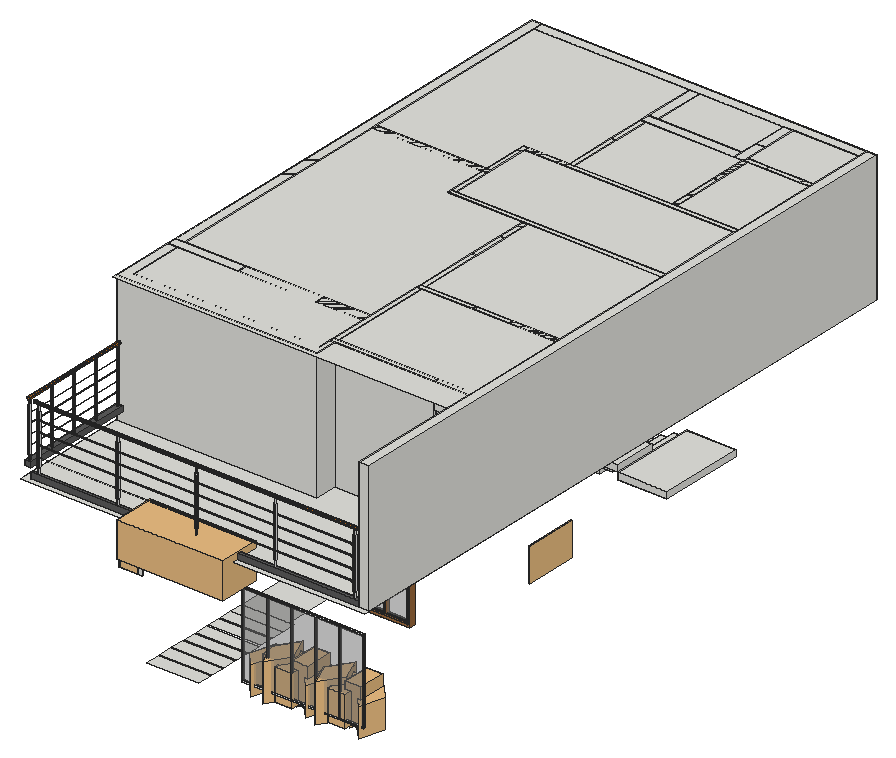
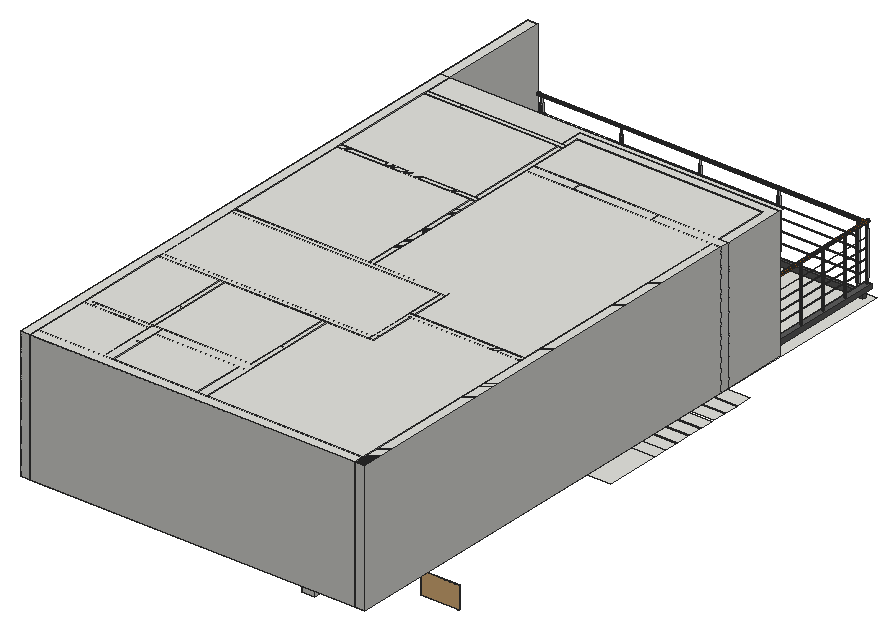
# SketchUp Ruby script. Lengths in inches.
U = 1.inch
M = Sketchup.active_model
def pt(a) = Geom::Point3d.new(a.map { |v| v * U })
def face(e, loops, mat)
  f = e.add_face(loops[0].map { |a| pt(a) })
  loops[1..].each { |l| e.add_face(l.map { |a| pt(a) }).erase! }
  f.material = f.back_material = mat if mat
  f
end
# faces: each face lists its corners as indices into pts; further lists are holes
def faces(e, pts, list, mat = nil) = list.each { |f| face(e, (f[0].is_a?(Array) ? f : [f]).map { |l| l.map { |i| pts[i] } }, mat) }
# xy, xz, yz: faces in a plane at the given z, y or x. An outline is a flat list of corners, or four numbers for a rectangle; further outlines are holes
def ring(l) = l.size == 4 ? [[l[0], l[1]], [l[2], l[1]], [l[2], l[3]], [l[0], l[3]]] : l.each_slice(2).to_a
def flat(e, list, mat, &to3) = list.each { |f| face(e, (f[0].is_a?(Array) ? f : [f]).map { |l| ring(l).map { |u, v| to3.(u, v) } }, mat) }
def xy(e, z, list, mat = nil) = flat(e, list, mat) { |x, y| [x, y, z] }
def xz(e, y, list, mat = nil) = flat(e, list, mat) { |x, z| [x, y, z] }
def yz(e, x, list, mat = nil) = flat(e, list, mat) { |y, z| [x, y, z] }
def lines(e, pts, list) = list.each { |a, b| e.add_line(pt(pts[a]), pt(pts[b])) }
# prism: a flat outline (further loops are holes) pulled along v
def prism(e, loops, v, mat = nil)
  f = face(e, loops, mat); d = Geom::Vector3d.new(v.map { |x| x * U })
  f.pushpull(f.normal.samedirection?(d) ? d.length : -d.length)
end
def box(e, o, s, mat = nil) = prism(e, [[o, [o[0] + s[0], o[1], o[2]], [o[0] + s[0], o[1] + s[1], o[2]], [o[0], o[1] + s[1], o[2]]]], [0, 0, s[2]], mat)
def at(x, y, z, deg = 0) = Geom::Transformation.translation(pt([x, y, z])) * Geom::Transformation.rotation(ORIGIN, Z_AXIS, deg.degrees)
def axes(o, x, y, z) = Geom::Transformation.new([*x, 0, *y, 0, *z, 0, *pt(o).to_a, 1])
def part(name) = M.definitions.add(name)
# library, detail: a bought-in or finely detailed component or shape, given as its bounding box
def library(name, o, s) = part(name).tap { |d| box(d.entities, o, s) }
def detail(e, o, s) = box(e.add_group.entities, o, s)
def put(e, d, t, mat = nil) = e.add_instance(d, t).tap { |i| i.material = mat if mat }
def group(e, t, mat = nil) = e.add_group.tap { |g| g.transformation = t; g.material = mat if mat }.entities
root = M.entities
M.materials.add("JJJ1").color = [238, 218, 183]
M.materials.add("MU TIGHI 6T67L 1").color = [235, 235, 235]
M.materials.add("Polis06_194").color = [79, 50, 36]
M.materials.add("Stone_A_200cm").color = [133, 133, 133]
M.materials.add("T ER5Y 565N 1").color = [201, 111, 22]
M.materials.add("T R72 56 8, 7 5U1").color = [25, 25, 25]
M.materials.add("[Color M00]").color = [255, 255, 255]
M.materials.add("[Color M09]").color = [0, 0, 0]
M.materials.add("[Translucent Glass Gray]").color = [128, 128, 128]
M.materials["[Translucent Glass Gray]"].alpha = 0.5
M.materials.add("[Translucent Glass Gray]1").color = [128, 128, 128]
M.materials["[Translucent Glass Gray]1"].alpha = 0.29
M.materials.add("[Translucent_Glass_Gray]").color = [128, 128, 128]
M.materials["[Translucent_Glass_Gray]"].alpha = 0.5
M.materials.add("[Wood Floor]").color = [155, 105, 61]
M.materials.add("wefsd tger 1").color = [92, 92, 92]
c1 = library("Group\#103",[-84.69,-90.07,-0.36],[176.51,175.13,171.4])
c2 = library("Areca palm plant",[0,0,0],[49.1,36.6,54.46])
c3 = part("Group\#23")
box(c3.entities,[0,0,0],[12.05,39.48,6])
c4 = library("Group\#130",[-7.34,-1.2,0],[38.67,35.81,49.04])
c5 = library("Group20\#1",[-20.81,-17.08,3.79],[39.86,39.43,37.51])
c6 = library("Group38\#2",[14.01,28.44,-23.43],[18.58,18.32,38.89])
c7 = part("W1")
xy(c7.entities,15,[[0,0,2,198]])
xy(c7.entities,102.0625,[[0,0,2,198]],"[Color M00]")
xz(c7.entities,0,[[0,15,2,102.0625]],"[Color M00]")
xz(c7.entities,198,[[0,15,2,102.0625]])
yz(c7.entities,0,[[0.84,16,39.43,101.0625],[40.28,16,78.87,101.0625],[79.71,16,118.3,101.0625],[119.14,16,157.73,101.0625],[158.58,16,197.16,101.0625]])
yz(c7.entities,0,[[[0,15,198,102.0625],[0.84,16,197.16,101.0625]],[39.43,16,40.28,101.0625],[78.87,16,79.71,101.0625],[118.3,16,119.14,101.0625],[157.73,16,158.58,101.0625]],"[Color M00]")
yz(c7.entities,2,[[0.84,16,39.43,101.0625],[40.28,16,78.87,101.0625],[79.71,16,118.3,101.0625],[119.14,16,157.73,101.0625],[158.58,16,197.16,101.0625]])
yz(c7.entities,2,[[[0,15,198,102.0625],[0.84,16,197.16,101.0625]],[39.43,16,40.28,101.0625],[78.87,16,79.71,101.0625],[118.3,16,119.14,101.0625],[157.73,16,158.58,101.0625]],"[Color M00]")
c8 = part("window full")
xy(c8.entities,0,[[0,0,14.17,66.54]])
xy(c8.entities,2.26,[[12.2,2.26,14.17,64.28]],"[Wood Floor]")
xy(c8.entities,2.36,[[0,2.36,1.97,64.17]],"[Wood Floor]")
xy(c8.entities,3.74,[[11.42,3.74,12.2,32.875],[11.42,33.66,12.2,62.79]],"[Wood Floor]")
xy(c8.entities,3.9375,[[1.97,3.9375,2.76,32.77],[1.97,33.76,2.76,62.6]],"[Wood Floor]")
xy(c8.entities,4.18,[[2.76,4.18,7.09,32.09],[7.09,4.18,11.42,32.09],[2.76,34.45,7.09,62.35],[7.09,34.45,11.42,62.35]],"[Wood Floor]")
xy(c8.entities,69.83,[[2.76,4.18,7.09,32.09],[7.09,32.09,11.42,34.45],[2.76,34.45,7.09,62.35]])
xy(c8.entities,69.83,[[7.09,4.18,11.42,32.09],[7.09,34.45,11.42,62.35]],"[Wood Floor]")
xy(c8.entities,70.08,[[1.97,3.9375,2.76,32.77],[1.97,33.76,2.76,62.6]])
xy(c8.entities,70.27,[[11.42,32.875,12.2,33.66]])
xy(c8.entities,70.27,[[11.42,3.74,12.2,32.875],[11.42,33.66,12.2,62.79]],"[Wood Floor]")
xy(c8.entities,71.65,[[0,2.36,1.97,64.17]])
xy(c8.entities,71.76,[[12.2,2.26,14.17,64.28]],"[Wood Floor]")
xy(c8.entities,74.02,[[0,0,14.17,66.54]],"[Wood Floor]")
xz(c8.entities,0,[[0,0,14.17,74.02]],"[Wood Floor]")
xz(c8.entities,2.26,[[12.2,2.26,14.17,71.76]],"[Wood Floor]")
xz(c8.entities,2.36,[[0,2.36,1.97,71.65]],"[Wood Floor]")
xz(c8.entities,3.74,[[11.42,3.74,12.2,70.27]],"[Wood Floor]")
xz(c8.entities,3.9375,[[1.97,3.9375,2.76,70.08]],"[Wood Floor]")
xz(c8.entities,4.18,[[2.76,4.18,7.09,69.83],[7.09,4.18,11.42,69.83]],"[Wood Floor]")
xz(c8.entities,32.09,[[2.76,4.18,11.42,69.83]],"[Wood Floor]")
xz(c8.entities,32.77,[[1.97,3.9375,2.76,70.08]],"[Wood Floor]")
xz(c8.entities,32.875,[[11.42,3.74,12.2,70.27]],"[Wood Floor]")
xz(c8.entities,33.66,[[11.42,3.74,12.2,47.88],[11.42,47.88,12.2,70.27]],"[Wood Floor]")
xz(c8.entities,33.76,[[1.97,3.9375,2.76,70.08]],"[Wood Floor]")
xz(c8.entities,34.45,[[2.76,4.18,11.42,69.83]],"[Wood Floor]")
xz(c8.entities,62.35,[[2.76,4.18,7.09,69.83],[7.09,4.18,11.42,69.83]],"[Wood Floor]")
xz(c8.entities,62.6,[[1.97,3.9375,2.76,70.08]],"[Wood Floor]")
xz(c8.entities,62.79,[[11.42,3.74,12.2,70.27]],"[Wood Floor]")
xz(c8.entities,64.17,[[0,2.36,1.97,71.65]],"[Wood Floor]")
xz(c8.entities,64.28,[[12.2,2.26,14.17,71.76]],"[Wood Floor]")
xz(c8.entities,66.54,[[0,0,14.17,74.02]],"[Wood Floor]")
yz(c8.entities,0,[[[0,0,66.54,74.02],[2.36,2.36,64.17,71.65]]],"[Wood Floor]")
yz(c8.entities,1.97,[[[2.36,2.36,64.17,71.65],[33.76,3.9375,62.6,70.08],[3.9375,3.9375,32.77,70.08]]],"[Wood Floor]")
yz(c8.entities,2.76,[[32.77,3.9375,33.76,4.18],[32.77,4.18,33.76,69.83],[32.77,69.83,33.76,70.08]])
yz(c8.entities,2.76,[[[3.9375,3.9375,32.77,70.08],[4.18,4.18,32.09,69.83]],[[33.76,3.9375,62.6,70.08],[34.45,4.18,62.35,69.83]]],"[Wood Floor]")
yz(c8.entities,7.09,[[4.18,4.18,62.35,69.83]],"[Translucent Glass Gray]")
yz(c8.entities,11.42,[[32.875,69.83,33.66,70.27]])
yz(c8.entities,11.42,[[[3.74,3.74,32.875,70.27],[4.18,4.18,32.09,69.83]],[[33.66,3.74,62.79,70.27],[34.45,4.18,62.35,69.83]]],"[Wood Floor]")
yz(c8.entities,12.2,[[[2.26,2.26,64.28,71.76],[3.74,3.74,32.875,70.27],[33.66,3.74,62.79,70.27]]],"[Wood Floor]")
yz(c8.entities,14.17,[[[0,0,66.54,74.02],[2.26,2.26,64.28,71.76]]],"[Wood Floor]")
p = [[11.42,32.875,70.27],[11.42,32.875,70.28]]
lines(c8.entities,p,[[0,1]])
c9 = library("Flat screen television",[0,1.41,1.14],[35.92,0.28,20.21])
c10 = library("TempSimLab_2015-06-11-13-14-41",[-24.54,-1.375,2.18],[48.7,1.34,30.98])
c11 = part("Group\#54")
prism(c11.entities,[[[0,39.5,0],[12,39.52,0],[12.05,0.02,0],[0.05,0,0]]],[0,0,6])
c12 = library("B_HOUSE",[0,0,0],[67.64,11.09,0.98])
c13 = library("Group\#92",[-9.3,-11.72,-5.59],[177.13,38.12,35])
c14 = part("Component\#28")
box(c14.entities,[0,0,0],[7.875,7.875,3.9375],"Stone_A_200cm")
c15 = part("Flush door")
xy(c15.entities,0,[[0,0,4.72,1.18],[0,34.25,4.72,35.43]],"Polis06_194")
xy(c15.entities,85.26,[[0,1.18,4.72,34.25]],"Polis06_194")
xy(c15.entities,86.61,[[0,0,4.72,35.43]],"Polis06_194")
xz(c15.entities,0,[[0,0,4.72,86.61]],"Polis06_194")
xz(c15.entities,1.18,[[0,0,2.36,85.26],[2.36,0,4.72,85.26]],"Polis06_194")
xz(c15.entities,34.25,[[0,0,4.72,85.26]],"Polis06_194")
xz(c15.entities,35.43,[[0,0,4.72,86.61]],"Polis06_194")
yz(c15.entities,0,[[0,0,1.18,86.61],[34.25,0,35.43,86.61],[1.18,85.26,34.25,86.61]],"Polis06_194")
yz(c15.entities,2.36,[[1.18,0,34.25,0,34.25,85.21,1.18,85.26]],"Polis06_194")
yz(c15.entities,4.72,[[0,0,1.18,86.61],[34.25,0,35.43,86.61],[1.18,85.26,34.25,86.61]],"Polis06_194")
c16 = part("Group\#68")
p = [[0,43.31,5.11],[2.95,43.31,0],[2.95,0,0],[0,0,5.11]]
faces(c16.entities,p,[[0,1,2,3]],"[Translucent_Glass_Gray]")
c17 = part("Vwntilation+window (2)")
put(c17.entities,c16,at(43.48,1.97,32.29))
put(c17.entities,c16,at(43.48,1.97,26.38))
put(c17.entities,c16,at(43.48,1.97,20.48))
put(c17.entities,c16,at(43.48,1.97,14.57))
put(c17.entities,c16,at(43.48,1.97,8.67))
put(c17.entities,c16,at(43.48,1.97,2.76))
g1 = group(c17.entities,at(43.48,0,0))
prism(g1,[[[1.97,47.24,39.37],[1.97,0,39.37],[1.97,0,0],[1.97,47.24,0]],[[1.97,45.28,1.97],[1.97,1.97,1.97],[1.97,1.97,37.4],[1.97,45.28,37.4]]],[-1.97,0,0])
c18 = part("Box01")
box(c18.entities,[-251.12,-5.93,-8.91],[582.61,12.27,8.91],"wefsd tger 1")
c19 = part("Box45")
box(c19.entities,[-240.91,-0.82,12.1],[2.44,1.82,74.48],"JJJ1")
c20 = part("Cylinder01")
prism(c20.entities,[[[328.21,-1.16,98.56],[328.21,-0.34,98.26],[328.21,0.53,98.26],[328.21,1.34,98.56],[328.21,2.01,99.11],[328.21,2.44,99.87],[328.21,2.59,100.72],[328.21,2.44,101.58],[328.21,2.01,102.33],[328.21,1.34,102.89],[328.21,0.53,103.18],[328.21,-0.34,103.18],[328.21,-1.16,102.89],[328.21,-1.82,102.33],[328.21,-2.25,101.58],[328.21,-2.41,100.72],[328.21,-2.25,99.87],[328.21,-1.82,99.11]]],[-576.3,0,0],"T ER5Y 565N 1")
c21 = part("Cylinder02")
prism(c21.entities,[[[-239.93,0.18,76.32],[-239.93,0.34,76.26],[-239.93,0.48,76.15],[-239.93,0.5625,75.99],[-239.93,0.59,75.82],[-239.93,0.5625,75.65],[-239.93,0.48,75.5],[-239.93,0.34,75.39],[-239.93,0.18,75.33],[-239.93,0.01,75.33],[-239.93,-0.16,75.39],[-239.93,-0.29,75.5],[-239.93,-0.375,75.65],[-239.93,-0.41,75.82],[-239.93,-0.375,75.99],[-239.93,-0.29,76.15],[-239.93,-0.16,76.26],[-239.93,0.01,76.32]]],[560.05,0,0],"T R72 56 8, 7 5U1")
c22 = part("Rectangle1")
prism(c22.entities,[[[-237.41,1.91,10.08],[-239.22,1.91,10.08],[-239.22,1.91,0.02],[-240.41,1.91,0.02],[-240.41,1.91,10.08],[-242.22,1.91,10.08],[-242.22,1.91,89.41],[-240.41,1.91,89.41],[-240.41,1.91,99.1875],[-239.22,1.91,99.1875],[-239.22,1.91,89.41],[-237.41,1.91,89.41]],[[-240.4375,1.91,85.68],[-240.4375,1.91,13.53],[-239.08,1.91,13.53],[-239.08,1.91,85.68]]],[0,-3.64,0],"MU TIGHI 6T67L 1")
c23 = part("skp243")
put(c23.entities,c18,at(0,0,0))
put(c23.entities,c19,at(0,0,0))
put(c23.entities,c20,at(0,0,0))
put(c23.entities,c21,at(0,0,0))
put(c23.entities,c22,at(0,0,0))
put(c23.entities,c21,at(0,0,-17.07))
put(c23.entities,c21,at(0,0,-35.38))
put(c23.entities,c21,at(0,0,-53.15))
put(c23.entities,c19,at(139.83,0,0))
put(c23.entities,c22,at(139.83,0,0))
put(c23.entities,c22,at(279.78,0,0))
put(c23.entities,c19,at(279.78,0,0))
put(c23.entities,c19,at(419.57,0,0))
put(c23.entities,c22,at(419.57,0,0))
put(c23.entities,c22,at(561.11,0,0))
put(c23.entities,c19,at(561.11,0,0))
c24 = part("Railing1 (1)")
put(c24.entities,c23,at(251.12,5.93,8.91))
c25 = part("Group\#49")
box(c25.entities,[0,0,0],[12.05,39.33,6])
xy(root,2,[[138.47,57,186.47,70.5],[138.47,72.5,186.47,84.5],[138.47,86.5,186.47,98.5],[138.47,100.5,186.47,112.5],[138.47,114.5,186.47,126.5],
  [138.47,128.5,186.47,140.5],[138.47,142.5,186.47,154.5],[138.47,154.5,186.47,166.5],[138.47,166.5,181.66,218]])
xy(root,120,[[28.97,48,346.97,638.5]])
put(root,c1,axes([304.91,79.66,5.45],[-0.04107,0.04465,0],[-0.02371,-0.07734,0],[0,0,0.0947]))
put(root,c1,axes([314.5,79.66,5.45],[-0.04107,0.04465,0],[-0.02371,-0.07734,0],[0,0,0.0947]))
put(root,c1,axes([291.89,79.66,5.45],[-0.04107,0.04465,0],[-0.02371,-0.07734,0],[0,0,0.0947]))
put(root,c1,axes([243.23,79.66,5.45],[-0.04107,0.04465,0],[-0.02371,-0.07734,0],[0,0,0.0947]))
put(root,c1,axes([256.25,79.66,5.45],[-0.04107,0.04465,0],[-0.02371,-0.07734,0],[0,0,0.0947]))
put(root,c1,axes([265.84,79.66,5.45],[-0.04107,0.04465,0],[-0.02371,-0.07734,0],[0,0,0.0947]))
put(root,c1,axes([280.11,77.63,5.47],[-0.06732,0.0732,0],[-0.03887,-0.12678,0],[0,0,0.15525]))
put(root,c1,axes([229.72,77.63,5.47],[-0.06732,0.0732,0],[-0.03887,-0.12678,0],[0,0,0.15525]))
put(root,c1,axes([328.77,77.63,5.47],[-0.06732,0.0732,0],[-0.03887,-0.12678,0],[0,0,0.15525]))
put(root,c2,axes([297.88,98.68,5.48],[-0.26854,-0.40516,0],[0.25322,-0.59523,0],[0,0,0.648]))
put(root,c2,axes([249.22,98.68,5.48],[-0.26854,-0.40516,0],[0.25322,-0.59523,0],[0,0,0.648]))
put(root,c3,at(196.65,447.38,6))
put(root,c4,axes([265.14,70.66,7.2],[0.37755,0,0],[0,0.711,0],[0,0,0.711]))
put(root,c4,axes([313.8,70.66,7.2],[0.37755,0,0],[0,0.711,0],[0,0,0.711]))
put(root,c5,axes([260.4,76.03,4.3],[0.40622,0,0],[0,0.765,0],[0,0,0.765]))
put(root,c5,axes([309.05,76.03,4.3],[0.40622,0,0],[0,0.765,0],[0,0,0.765]))
put(root,c6,axes([221.625,96.8,25.35],[0,-0.79632,0],[0.45245,0,0],[0,0,0.77243]))
put(root,c6,axes([270.28,96.8,25.35],[0,-0.79632,0],[0.45245,0,0],[0,0,0.77243]))
put(root,c3,at(208.7,447.38,12))
put(root,c7,axes([222.18,64.3,0],[0,-0.9,0],[0.56673,0,0],[0,0,0.9]),"[Translucent Glass Gray]1")
put(root,c3,at(220.75,447.38,18))
put(root,c3,at(232.8,447.38,24))
put(root,c3,at(244.85,447.38,30))
put(root,c8,axes([291.92,168.52,36],[0,0.4275,0],[-0.72142,0,0],[0,0,0.64851]))
put(root,c3,at(256.9,447.38,36))
put(root,c3,at(268.95,447.38,42))
put(root,c9,at(188.82,267,42.23,90))
put(root,c9,at(94.34,493.52,45.0625,180))
put(root,c3,at(281,447.38,48))
put(root,c10,at(338.01,274.3125,50.51,-90))
g2 = group(root,at(293.05,407.86,54))
box(g2,[0,0,0],[45.375,79,6])
put(root,c11,at(281,407.86,60))
put(root,c11,at(269,407.86,66))
put(root,c11,at(257,407.86,72))
g3 = group(root,at(146.24,51.15,76.77))
box(g3,[-28.68,0,0],[21.64,0.79,11.8125])
put(root,c12,axes([118.79,51.15,77.42],[0.24123,0,0],[0,0,0.9088],[0,-0.64,0]),"[Color M09]")
put(root,c11,at(245,407.86,78))
put(root,c11,at(233,407.86,84))
put(root,c11,at(221,407.86,90))
put(root,c13,axes([132.7,48,98.23],[0.55,0,0],[0,1,0],[0,0,0.94148]))
put(root,c11,at(209,407.86,96))
g4 = group(root,at(115.85,487,0))
box(g4,[0,0,96],[40,4.5,24])
g5 = group(root,at(273.47,493.55,0))
box(g5,[0,0,96],[4.5,32.16,24])
put(root,c14,axes([140.28,49.97,100.39],[0.55,0,0],[0,1,0],[0,0,1]))
put(root,c14,axes([216.08,49.97,100.39],[0.55,0,0],[0,1,0],[0,0,1]))
put(root,c11,at(197,407.86,102))
put(root,c11,at(185,407.85,108))
g6 = group(root,at(28.97,53,120))
xy(g6,0,[[[0,0,309,576.5],[153,437.37,157.5,437.5]],[153,437.37,157.5,437.5]])
xy(g6,120,[[0,101.55,318,585.5]])
put(g6,c15,axes([111.86,354.25,0],[0.7,0,0],[0,1.00894,0],[0,0,1.10836]))
put(g6,c15,axes([111.86,430.25,0],[0.7,0,0],[0,-1.00894,0],[0,0,1.10836]))
put(g6,c15,axes([300.53,519.5,0],[0,0.7,0],[-0.9075,0,0],[0,0,1.10836]))
put(g6,c17,axes([277,179.91,60],[0,-1.16,0],[0.67733,0,0],[0,0,0.92]))
put(g6,c17,axes([197.55,544.5,60],[1,0,0],[0,0.67733,0],[0,0,1]))
put(g6,c8,axes([137.1875,165,36],[0,0.4275,0],[-1.08213,0,0],[0,0,0.64851]))
put(g6,c15,axes([247.5,485.52,0],[0.7,0,0],[0,0.9075,0],[0,0,1.10836]))
put(g6,c15,axes([153,485.52,0],[0.7,0,0],[0,0.9075,0],[0,0,1.10836]))
put(g6,c15,axes([180.5,290.47,0],[0.7,0,0],[0,0.9075,0],[0,0,1.10836]))
put(g6,c15,axes([265.35,227,0],[0,0.7,0],[-0.9075,0,0],[0,0,1.10836]))
put(g6,c24,axes([6.04,0,0],[0.52,0,0],[0,0.26,0],[0,0,0.58]))
put(g6,c24,axes([0,106,8.91],[0,-0.18194,0],[0.49244,0,0],[0,0,0.51123]))
g7 = group(g6,at(0,106,0))
prism(g7,[[[185,0,0],[0,0,0],[0,59,0],[9,59,0],[9,9,0],[180.5,9,0],[180.5,20.5,0],[185,20.5,0]]],[0,0,120])
g8 = group(g6,at(65.1875,165,0))
box(g8,[0,0,0],[72,9,36])
box(g8,[0,0,84],[72,9,36])
p = [[0,9,36],[0,9,84],[72,9,36],[72,9,84]]
lines(g8,p,[[0,1],[2,3]])
g9 = group(g6,at(180.5,126.5,0))
prism(g9,[[[4.5,0,0],[0,0,0],[0,4.5,0],[4.5,4.5,0],[96.5,4.5,0],[96.5,0,0]]],[0,0,120])
g10 = group(g6,at(9,390,0))
box(g10,[0,0,0],[106.17,4.5,120])
g11 = group(g6,at(0,165,0))
prism(g11,[[[65.1875,9,0],[65.1875,0,0],[9,0,0],[0,0,0],[0,9,0],[9,9,0]]],[0,0,120])
g12 = group(g6,at(137.1875,165,0))
box(g12,[0,0,0],[43.3125,9,120])
g13 = group(g6,at(239.5,519.5,0))
prism(g13,[[[9,4.5,0],[9,0,0],[0,0,0],[0,8.85,0],[0,25,0],[9,25,0]]],[0,0,120])
g14 = group(g6,at(153,519.5,0))
box(g14,[0,0,0],[86.5,8.85,120])
g15 = group(g6,at(153,528.5,0))
box(g15,[0,0,0],[9,48,120])
g16 = group(g6,at(309,0,0))
prism(g16,[[[0,576.5,0],[0,585.5,0],[9,585.5,0],[9,0,0],[0,0,0],[0,126.5,0],[0,131,0],[0,227,0],[0,231.5,0],[0,349.55,0],[0,354,0],[0,432.8125,0],[0,437.5,0],[0,519.5,0],[0,524,0]]],[0,0,120])
g17 = group(g6,at(247.5,437.5,0))
box(g17,[0,0,0],[4.5,48.02,120])
g18 = group(g6,at(153,437.5,0))
box(g18,[0,0,0],[4.5,48.02,120])
g19 = group(g6,at(180.5,131,0))
prism(g19,[[[0,0,0],[0,34,0],[0,43,0],[0,96,0],[4.5,96,0],[4.5,0,0]]],[0,0,120])
g20 = group(g6,at(0,174,0))
prism(g20,[[[0,0,0],[0,411.5,0],[9,411.5,0],[9,402.5,0],[9,220.5,0],[9,216,0],[9,0,0]]],[0,0,120])
g21 = group(g6,at(115.17,432.8125,0))
prism(g21,[[[193.83,0,0],[0,0,0],[0,4.49,0],[0,4.6875,0],[37.83,4.6875,0],[37.83,4.55,0],[42.33,4.55,0],[42.33,4.6875,0],[132.33,4.6875,0],[136.83,4.6875,0],[193.83,4.6875,0]]],[0,0,120])
g22 = group(g6,at(9,576.5,0))
prism(g22,[[[0,9,0],[300,9,0],[300,0,0],[239.5,0,0],[230.5,0,0],[153,0,0],[144,0,0],[0,0,0]]],[0,0,120])
g23 = group(g6,at(180.5,231.5,0))
box(g23,[0,0,0],[4.5,58.97,120])
g24 = group(g6,at(110.67,430.25,0))
prism(g24,[[[0,7.06,0],[4.5,7.06,0],[4.5,2.5625,0],[4.5,0,0],[0,0,0]]],[0,0,120])
g25 = group(g6,at(180.5,322.77,0))
box(g25,[0,0,0],[4.5,26.73,120])
put(g6,c25,at(203.82,393.48,24))
put(g6,c25,at(155.625,393.48,0))
put(g6,c25,at(227.92,393.48,36))
put(g6,c25,at(191.77,393.48,18))
g26 = group(g6,at(264.07,354,54))
box(g26,[0,0,0],[45.28,78.8125,6])
g27 = group(g6,at(110.67,349.55,0))
box(g27,[0,0,0],[198.33,4.45,120])
put(g6,c25,at(252.02,354,60))
put(g6,c25,at(191.77,354,90))
put(g6,c25,at(167.67,393.48,6))
put(g6,c25,at(239.97,393.48,42))
put(g6,c25,at(215.875,354,78))
put(g6,c25,at(155.625,354,108))
put(g6,c25,at(167.67,354,102))
put(g6,c25,at(215.875,393.48,30))
put(g6,c25,at(179.72,393.48,12))
put(g6,c25,at(252.02,393.48,48))
put(g6,c25,at(227.92,354,72))
g28 = group(g6,at(265.51,227,0))
box(g28,[0,0,0],[43.49,4.5,120])
put(g6,c25,at(203.82,354,84))
g29 = group(g6,at(180.5,227,0))
prism(g29,[[[4.5,0,0],[0,0,0],[0,4.5,0],[4.5,4.5,0],[52.7,4.5,0],[52.7,0,0]]],[0,0,120])
put(g6,c25,at(179.72,354,96))
put(g6,c25,at(239.97,354,66))
g30 = group(g6,at(239.5,544.5,0))
box(g30,[0,0,0],[9,32,60])
box(g30,[0,0,96],[9,32,24])
p = [[9,0,60],[9,0,96],[9,32,60],[9,32,96]]
lines(g30,p,[[0,1],[2,3]])
g31 = group(g6,at(268.38,519.5,0))
box(g31,[0,0,96],[32,4.5,24])
g32 = group(g6,at(233.2,227,0))
box(g32,[0,0,96],[32.31,4.5,24])
g33 = group(g6,at(110.67,354,0))
box(g33,[0,0,96],[4.5,36,24])
g34 = group(g6,at(277,126.5,0))
box(g34,[0,0,0],[32,4.5,60])
box(g34,[0,0,96],[32,4.5,24])
p = [[0,4.5,60],[0,4.5,96],[32,4.5,60],[32,4.5,96]]
lines(g34,p,[[0,1],[2,3]])
g35 = group(g6,at(247.5,485.52,0))
box(g35,[0,0,96],[4.5,33.98,24])
g36 = group(g6,at(248.5,519.5,0))
box(g36,[0,0,0],[19.88,4.5,120])
g37 = group(g6,at(300.38,519.5,0))
box(g37,[0,0,0],[8.62,4.5,120])
g38 = group(g6,at(153,485.52,0))
box(g38,[0,0,96],[4.85,33.98,24])
g39 = group(g6,at(110.67,394.5,0))
box(g39,[0,0,96],[4.5,35.75,24])
g40 = group(g6,at(180.5,290.47,0))
box(g40,[0,0,96],[4.85,32.31,24])
